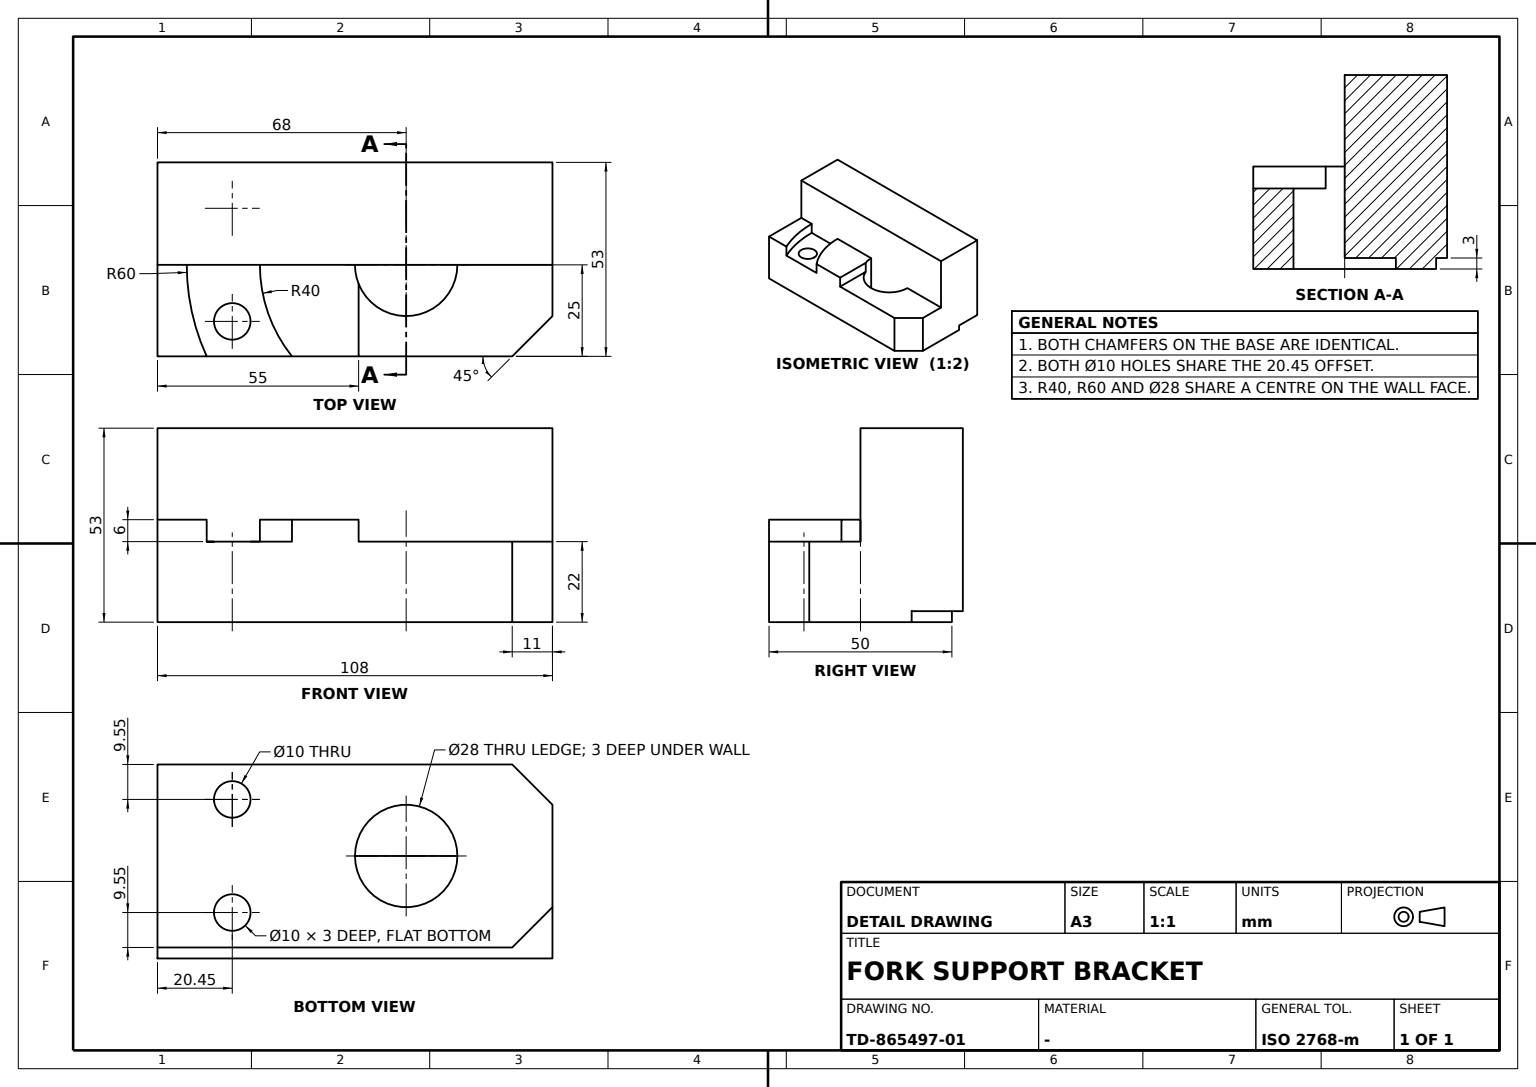
ISO-10303-21;
HEADER;
FILE_DESCRIPTION((''),'2;1');
FILE_NAME('','',(''),(''),'','','');
FILE_SCHEMA(('AUTOMOTIVE_DESIGN'));
ENDSEC;
DATA;
#1=APPLICATION_CONTEXT('');
#2=PRODUCT_CONTEXT('',#1,'mechanical');
#3=PRODUCT('','','',(#2));
#4=PRODUCT_DEFINITION_FORMATION('','',#3);
#5=PRODUCT_DEFINITION_CONTEXT('',#1,'design');
#6=PRODUCT_DEFINITION('','',#4,#5);
#7=PRODUCT_DEFINITION_SHAPE('','',#6);
#8=(LENGTH_UNIT()NAMED_UNIT(*)SI_UNIT(.MILLI.,.METRE.));
#9=(NAMED_UNIT(*)PLANE_ANGLE_UNIT()SI_UNIT($,.RADIAN.));
#10=(NAMED_UNIT(*)SI_UNIT($,.STERADIAN.)SOLID_ANGLE_UNIT());
#11=UNCERTAINTY_MEASURE_WITH_UNIT(LENGTH_MEASURE(1.E-05),#8,'distance_accuracy_value','');
#12=(GEOMETRIC_REPRESENTATION_CONTEXT(3)GLOBAL_UNCERTAINTY_ASSIGNED_CONTEXT((#11))GLOBAL_UNIT_ASSIGNED_CONTEXT((#8,#9,#10))REPRESENTATION_CONTEXT('',''));
#13=CARTESIAN_POINT('',(0.,0.,53.));
#14=VERTEX_POINT('',#13);
#15=CARTESIAN_POINT('',(0.,28.,53.));
#16=VERTEX_POINT('',#15);
#17=CARTESIAN_POINT('',(0.,14.,53.));
#18=DIRECTION('',(0.,1.,0.));
#19=VECTOR('',#18,1000.);
#20=LINE('',#17,#19);
#21=EDGE_CURVE('',#14,#16,#20,.T.);
#22=ORIENTED_EDGE('',*,*,#21,.T.);
#23=CARTESIAN_POINT('',(-108.,28.,53.));
#24=VERTEX_POINT('',#23);
#25=CARTESIAN_POINT('',(-54.,28.,53.));
#26=DIRECTION('',(-1.,0.,0.));
#27=VECTOR('',#26,1000.);
#28=LINE('',#25,#27);
#29=EDGE_CURVE('',#16,#24,#28,.T.);
#30=ORIENTED_EDGE('',*,*,#29,.T.);
#31=CARTESIAN_POINT('',(-108.,0.,53.));
#32=VERTEX_POINT('',#31);
#33=CARTESIAN_POINT('',(-108.,14.,53.));
#34=DIRECTION('',(0.,-1.,0.));
#35=VECTOR('',#34,1000.);
#36=LINE('',#33,#35);
#37=EDGE_CURVE('',#24,#32,#36,.T.);
#38=ORIENTED_EDGE('',*,*,#37,.T.);
#39=CARTESIAN_POINT('',(-54.,0.,53.));
#40=DIRECTION('',(1.,0.,0.));
#41=VECTOR('',#40,1000.);
#42=LINE('',#39,#41);
#43=EDGE_CURVE('',#32,#14,#42,.T.);
#44=ORIENTED_EDGE('',*,*,#43,.T.);
#45=EDGE_LOOP('',(#22,#30,#38,#44));
#46=FACE_OUTER_BOUND('',#45,.T.);
#47=DIRECTION('',(0.,0.,1.));
#48=AXIS2_PLACEMENT_3D('',#15,#47,#26);
#49=PLANE('',#48);
#50=ADVANCED_FACE('',(#46),#49,.T.);
#51=CARTESIAN_POINT('',(-53.,-5.196152,28.));
#52=VERTEX_POINT('',#51);
#53=CARTESIAN_POINT('',(-53.,-25.,28.));
#54=VERTEX_POINT('',#53);
#55=CARTESIAN_POINT('',(-53.,-15.098076,28.));
#56=LINE('',#55,#35);
#57=EDGE_CURVE('',#52,#54,#56,.T.);
#58=ORIENTED_EDGE('',*,*,#57,.F.);
#59=CARTESIAN_POINT('',(-54.,0.,28.));
#60=VERTEX_POINT('',#59);
#61=CARTESIAN_POINT('',(-40.,0.,28.));
#62=AXIS2_PLACEMENT_3D('',#61,#47,#40);
#63=CIRCLE('',#62,14.);
#64=EDGE_CURVE('',#60,#52,#63,.T.);
#65=ORIENTED_EDGE('',*,*,#64,.F.);
#66=CARTESIAN_POINT('',(-80.,0.,28.));
#67=VERTEX_POINT('',#66);
#68=CARTESIAN_POINT('',(-67.,0.,28.));
#69=LINE('',#68,#27);
#70=EDGE_CURVE('',#60,#67,#69,.T.);
#71=ORIENTED_EDGE('',*,*,#70,.T.);
#72=CARTESIAN_POINT('',(-71.22499,-25.,28.));
#73=VERTEX_POINT('',#72);
#74=DIRECTION('',(0.,0.,-1.));
#75=AXIS2_PLACEMENT_3D('',#61,#74,#40);
#76=CIRCLE('',#75,40.);
#77=EDGE_CURVE('',#73,#67,#76,.T.);
#78=ORIENTED_EDGE('',*,*,#77,.F.);
#79=CARTESIAN_POINT('',(-62.112495,-25.,28.));
#80=LINE('',#79,#41);
#81=EDGE_CURVE('',#73,#54,#80,.T.);
#82=ORIENTED_EDGE('',*,*,#81,.T.);
#83=EDGE_LOOP('',(#58,#65,#71,#78,#82));
#84=FACE_OUTER_BOUND('',#83,.T.);
#85=CARTESIAN_POINT('',(0.,0.,28.));
#86=AXIS2_PLACEMENT_3D('',#85,#74,#26);
#87=PLANE('',#86);
#88=ADVANCED_FACE('',(#84),#87,.F.);
#89=CARTESIAN_POINT('',(-108.,25.,3.));
#90=VERTEX_POINT('',#89);
#91=CARTESIAN_POINT('',(-11.,25.,3.));
#92=VERTEX_POINT('',#91);
#93=CARTESIAN_POINT('',(-59.5,25.,3.));
#94=LINE('',#93,#41);
#95=EDGE_CURVE('',#90,#92,#94,.T.);
#96=ORIENTED_EDGE('',*,*,#95,.F.);
#97=CARTESIAN_POINT('',(-108.,28.,3.));
#98=VERTEX_POINT('',#97);
#99=CARTESIAN_POINT('',(-108.,26.5,3.));
#100=LINE('',#99,#35);
#101=EDGE_CURVE('',#98,#90,#100,.T.);
#102=ORIENTED_EDGE('',*,*,#101,.F.);
#103=CARTESIAN_POINT('',(0.,28.,3.));
#104=VERTEX_POINT('',#103);
#105=CARTESIAN_POINT('',(-54.,28.,3.));
#106=LINE('',#105,#27);
#107=EDGE_CURVE('',#104,#98,#106,.T.);
#108=ORIENTED_EDGE('',*,*,#107,.F.);
#109=CARTESIAN_POINT('',(0.,14.,3.));
#110=VERTEX_POINT('',#109);
#111=CARTESIAN_POINT('',(0.,21.,3.));
#112=LINE('',#111,#19);
#113=EDGE_CURVE('',#110,#104,#112,.T.);
#114=ORIENTED_EDGE('',*,*,#113,.F.);
#115=CARTESIAN_POINT('',(-5.5,19.5,3.));
#116=DIRECTION('',(-0.707106781,0.707106781,0.));
#117=VECTOR('',#116,1000.);
#118=LINE('',#115,#117);
#119=EDGE_CURVE('',#110,#92,#118,.T.);
#120=ORIENTED_EDGE('',*,*,#119,.T.);
#121=EDGE_LOOP('',(#96,#102,#108,#114,#120));
#122=FACE_OUTER_BOUND('',#121,.T.);
#123=AXIS2_PLACEMENT_3D('',#103,#47,#26);
#124=PLANE('',#123);
#125=ADVANCED_FACE('',(#122),#124,.F.);
#126=CARTESIAN_POINT('',(-92.552826,15.45085,0.));
#127=VERTEX_POINT('',#126);
#128=CARTESIAN_POINT('',(-82.552826,15.45085,0.));
#129=VERTEX_POINT('',#128);
#130=CARTESIAN_POINT('',(-87.552826,15.45085,0.));
#131=AXIS2_PLACEMENT_3D('',#130,#47,#40);
#132=CIRCLE('',#131,5.);
#133=EDGE_CURVE('',#127,#129,#132,.T.);
#134=ORIENTED_EDGE('',*,*,#133,.T.);
#135=EDGE_CURVE('',#129,#127,#132,.T.);
#136=ORIENTED_EDGE('',*,*,#135,.T.);
#137=EDGE_LOOP('',(#134,#136));
#138=FACE_BOUND('',#137,.T.);
#139=CARTESIAN_POINT('',(-54.,0.,0.));
#140=VERTEX_POINT('',#139);
#141=CARTESIAN_POINT('',(-26.,0.,0.));
#142=VERTEX_POINT('',#141);
#143=CARTESIAN_POINT('',(-40.,0.,0.));
#144=AXIS2_PLACEMENT_3D('',#143,#47,#40);
#145=CIRCLE('',#144,14.);
#146=EDGE_CURVE('',#140,#142,#145,.T.);
#147=ORIENTED_EDGE('',*,*,#146,.T.);
#148=EDGE_CURVE('',#142,#140,#145,.T.);
#149=ORIENTED_EDGE('',*,*,#148,.T.);
#150=EDGE_LOOP('',(#147,#149));
#151=FACE_BOUND('',#150,.T.);
#152=CARTESIAN_POINT('',(-108.,-25.,0.));
#153=VERTEX_POINT('',#152);
#154=CARTESIAN_POINT('',(-108.,25.,0.));
#155=VERTEX_POINT('',#154);
#156=CARTESIAN_POINT('',(-108.,0.,0.));
#157=LINE('',#156,#19);
#158=EDGE_CURVE('',#153,#155,#157,.T.);
#159=ORIENTED_EDGE('',*,*,#158,.T.);
#160=CARTESIAN_POINT('',(-11.,25.,0.));
#161=VERTEX_POINT('',#160);
#162=CARTESIAN_POINT('',(-59.5,25.,0.));
#163=LINE('',#162,#27);
#164=EDGE_CURVE('',#161,#155,#163,.T.);
#165=ORIENTED_EDGE('',*,*,#164,.F.);
#166=CARTESIAN_POINT('',(0.,14.,0.));
#167=VERTEX_POINT('',#166);
#168=CARTESIAN_POINT('',(-5.5,19.5,0.));
#169=LINE('',#168,#117);
#170=EDGE_CURVE('',#167,#161,#169,.T.);
#171=ORIENTED_EDGE('',*,*,#170,.F.);
#172=CARTESIAN_POINT('',(0.,-14.,0.));
#173=VERTEX_POINT('',#172);
#174=CARTESIAN_POINT('',(0.,0.,0.));
#175=LINE('',#174,#19);
#176=EDGE_CURVE('',#173,#167,#175,.T.);
#177=ORIENTED_EDGE('',*,*,#176,.F.);
#178=CARTESIAN_POINT('',(-11.,-25.,0.));
#179=VERTEX_POINT('',#178);
#180=CARTESIAN_POINT('',(-5.5,-19.5,0.));
#181=DIRECTION('',(0.707106781,0.707106781,0.));
#182=VECTOR('',#181,1000.);
#183=LINE('',#180,#182);
#184=EDGE_CURVE('',#179,#173,#183,.T.);
#185=ORIENTED_EDGE('',*,*,#184,.F.);
#186=CARTESIAN_POINT('',(-59.5,-25.,0.));
#187=LINE('',#186,#27);
#188=EDGE_CURVE('',#179,#153,#187,.T.);
#189=ORIENTED_EDGE('',*,*,#188,.T.);
#190=EDGE_LOOP('',(#159,#165,#171,#177,#185,#189));
#191=FACE_OUTER_BOUND('',#190,.T.);
#192=CARTESIAN_POINT('',(-82.552826,-15.45085,0.));
#193=VERTEX_POINT('',#192);
#194=CARTESIAN_POINT('',(-92.552826,-15.45085,0.));
#195=VERTEX_POINT('',#194);
#196=CARTESIAN_POINT('',(-87.552826,-15.45085,0.));
#197=AXIS2_PLACEMENT_3D('',#196,#47,#40);
#198=CIRCLE('',#197,5.);
#199=EDGE_CURVE('',#193,#195,#198,.T.);
#200=ORIENTED_EDGE('',*,*,#199,.T.);
#201=EDGE_CURVE('',#195,#193,#198,.T.);
#202=ORIENTED_EDGE('',*,*,#201,.T.);
#203=EDGE_LOOP('',(#200,#202));
#204=FACE_BOUND('',#203,.T.);
#205=AXIS2_PLACEMENT_3D('',#156,#47,#40);
#206=PLANE('',#205);
#207=ADVANCED_FACE('',(#138,#151,#191,#204),#206,.F.);
#208=ORIENTED_EDGE('',*,*,#95,.T.);
#209=CARTESIAN_POINT('',(-11.,25.,1.5));
#210=VECTOR('',#74,1000.);
#211=LINE('',#209,#210);
#212=EDGE_CURVE('',#92,#161,#211,.T.);
#213=ORIENTED_EDGE('',*,*,#212,.T.);
#214=ORIENTED_EDGE('',*,*,#164,.T.);
#215=CARTESIAN_POINT('',(-108.,25.,1.5));
#216=VECTOR('',#47,1000.);
#217=LINE('',#215,#216);
#218=EDGE_CURVE('',#155,#90,#217,.T.);
#219=ORIENTED_EDGE('',*,*,#218,.T.);
#220=EDGE_LOOP('',(#208,#213,#214,#219));
#221=FACE_OUTER_BOUND('',#220,.T.);
#222=CARTESIAN_POINT('',(0.,25.,0.));
#223=AXIS2_PLACEMENT_3D('',#222,#18,#26);
#224=PLANE('',#223);
#225=ADVANCED_FACE('',(#221),#224,.T.);
#226=CARTESIAN_POINT('',(-82.552826,15.45085,3.));
#227=VERTEX_POINT('',#226);
#228=CARTESIAN_POINT('',(-92.552826,15.45085,3.));
#229=VERTEX_POINT('',#228);
#230=CARTESIAN_POINT('',(-87.552826,15.45085,3.));
#231=AXIS2_PLACEMENT_3D('',#230,#47,#26);
#232=CIRCLE('',#231,5.);
#233=EDGE_CURVE('',#227,#229,#232,.T.);
#234=ORIENTED_EDGE('',*,*,#233,.T.);
#235=CARTESIAN_POINT('',(-92.552826,15.45085,10.34));
#236=LINE('',#235,#210);
#237=EDGE_CURVE('',#229,#127,#236,.T.);
#238=ORIENTED_EDGE('',*,*,#237,.T.);
#239=ORIENTED_EDGE('',*,*,#135,.F.);
#240=CARTESIAN_POINT('',(-82.552826,15.45085,10.34));
#241=LINE('',#240,#210);
#242=EDGE_CURVE('',#227,#129,#241,.T.);
#243=ORIENTED_EDGE('',*,*,#242,.F.);
#244=EDGE_LOOP('',(#234,#238,#239,#243));
#245=FACE_OUTER_BOUND('',#244,.T.);
#246=CARTESIAN_POINT('',(-87.552826,15.45085,10.34));
#247=AXIS2_PLACEMENT_3D('',#246,#74,#40);
#248=CYLINDRICAL_SURFACE('',#247,5.);
#249=ADVANCED_FACE('',(#245),#248,.F.);
#250=CARTESIAN_POINT('',(-26.,0.,3.));
#251=VERTEX_POINT('',#250);
#252=CARTESIAN_POINT('',(-54.,0.,3.));
#253=VERTEX_POINT('',#252);
#254=CARTESIAN_POINT('',(-40.,0.,3.));
#255=AXIS2_PLACEMENT_3D('',#254,#47,#26);
#256=CIRCLE('',#255,14.);
#257=EDGE_CURVE('',#251,#253,#256,.T.);
#258=ORIENTED_EDGE('',*,*,#257,.F.);
#259=LINE('',#254,#41);
#260=EDGE_CURVE('',#253,#251,#259,.T.);
#261=ORIENTED_EDGE('',*,*,#260,.F.);
#262=EDGE_LOOP('',(#258,#261));
#263=FACE_OUTER_BOUND('',#262,.T.);
#264=ADVANCED_FACE('',(#263),#124,.F.);
#265=CARTESIAN_POINT('',(-53.,-25.,22.));
#266=VERTEX_POINT('',#265);
#267=CARTESIAN_POINT('',(-53.,-25.,25.));
#268=LINE('',#267,#210);
#269=EDGE_CURVE('',#54,#266,#268,.T.);
#270=ORIENTED_EDGE('',*,*,#269,.F.);
#271=ORIENTED_EDGE('',*,*,#81,.F.);
#272=CARTESIAN_POINT('',(-71.22499,-25.,22.));
#273=VERTEX_POINT('',#272);
#274=CARTESIAN_POINT('',(-71.22499,-25.,25.));
#275=LINE('',#274,#210);
#276=EDGE_CURVE('',#73,#273,#275,.T.);
#277=ORIENTED_EDGE('',*,*,#276,.T.);
#278=CARTESIAN_POINT('',(-94.543561,-25.,22.));
#279=VERTEX_POINT('',#278);
#280=CARTESIAN_POINT('',(-82.884275,-25.,22.));
#281=LINE('',#280,#41);
#282=EDGE_CURVE('',#279,#273,#281,.T.);
#283=ORIENTED_EDGE('',*,*,#282,.F.);
#284=CARTESIAN_POINT('',(-94.543561,-25.,28.));
#285=VERTEX_POINT('',#284);
#286=CARTESIAN_POINT('',(-94.543561,-25.,25.));
#287=LINE('',#286,#210);
#288=EDGE_CURVE('',#285,#279,#287,.T.);
#289=ORIENTED_EDGE('',*,*,#288,.F.);
#290=CARTESIAN_POINT('',(-108.,-25.,28.));
#291=VERTEX_POINT('',#290);
#292=CARTESIAN_POINT('',(-101.27178,-25.,28.));
#293=LINE('',#292,#41);
#294=EDGE_CURVE('',#291,#285,#293,.T.);
#295=ORIENTED_EDGE('',*,*,#294,.F.);
#296=CARTESIAN_POINT('',(-108.,-25.,14.));
#297=LINE('',#296,#216);
#298=EDGE_CURVE('',#153,#291,#297,.T.);
#299=ORIENTED_EDGE('',*,*,#298,.F.);
#300=ORIENTED_EDGE('',*,*,#188,.F.);
#301=CARTESIAN_POINT('',(-11.,-25.,22.));
#302=VERTEX_POINT('',#301);
#303=CARTESIAN_POINT('',(-11.,-25.,11.));
#304=LINE('',#303,#210);
#305=EDGE_CURVE('',#302,#179,#304,.T.);
#306=ORIENTED_EDGE('',*,*,#305,.F.);
#307=CARTESIAN_POINT('',(-32.,-25.,22.));
#308=LINE('',#307,#41);
#309=EDGE_CURVE('',#266,#302,#308,.T.);
#310=ORIENTED_EDGE('',*,*,#309,.F.);
#311=EDGE_LOOP('',(#270,#271,#277,#283,#289,#295,#299,#300,#306,#310));
#312=FACE_OUTER_BOUND('',#311,.T.);
#313=CARTESIAN_POINT('',(0.,-25.,0.));
#314=AXIS2_PLACEMENT_3D('',#313,#18,#26);
#315=PLANE('',#314);
#316=ADVANCED_FACE('',(#312),#315,.F.);
#317=CARTESIAN_POINT('',(0.,-14.,22.));
#318=VERTEX_POINT('',#317);
#319=CARTESIAN_POINT('',(0.,-14.,11.));
#320=LINE('',#319,#210);
#321=EDGE_CURVE('',#318,#173,#320,.T.);
#322=ORIENTED_EDGE('',*,*,#321,.F.);
#323=CARTESIAN_POINT('',(-5.5,-19.5,22.));
#324=DIRECTION('',(-0.707106781,-0.707106781,0.));
#325=VECTOR('',#324,1000.);
#326=LINE('',#323,#325);
#327=EDGE_CURVE('',#318,#302,#326,.T.);
#328=ORIENTED_EDGE('',*,*,#327,.T.);
#329=ORIENTED_EDGE('',*,*,#305,.T.);
#330=ORIENTED_EDGE('',*,*,#184,.T.);
#331=EDGE_LOOP('',(#322,#328,#329,#330));
#332=FACE_OUTER_BOUND('',#331,.T.);
#333=CARTESIAN_POINT('',(-11.,-25.,-5.6));
#334=AXIS2_PLACEMENT_3D('',#333,#116,#47);
#335=PLANE('',#334);
#336=ADVANCED_FACE('',(#332),#335,.F.);
#337=ORIENTED_EDGE('',*,*,#242,.T.);
#338=ORIENTED_EDGE('',*,*,#133,.F.);
#339=ORIENTED_EDGE('',*,*,#237,.F.);
#340=EDGE_CURVE('',#229,#227,#232,.T.);
#341=ORIENTED_EDGE('',*,*,#340,.T.);
#342=EDGE_LOOP('',(#337,#338,#339,#341));
#343=FACE_OUTER_BOUND('',#342,.T.);
#344=ADVANCED_FACE('',(#343),#248,.F.);
#345=CARTESIAN_POINT('',(-100.,0.,22.));
#346=VERTEX_POINT('',#345);
#347=CARTESIAN_POINT('',(-100.,0.,28.));
#348=VERTEX_POINT('',#347);
#349=CARTESIAN_POINT('',(-100.,0.,25.));
#350=LINE('',#349,#216);
#351=EDGE_CURVE('',#346,#348,#350,.T.);
#352=ORIENTED_EDGE('',*,*,#351,.T.);
#353=CIRCLE('',#62,60.);
#354=EDGE_CURVE('',#348,#285,#353,.T.);
#355=ORIENTED_EDGE('',*,*,#354,.T.);
#356=ORIENTED_EDGE('',*,*,#288,.T.);
#357=CARTESIAN_POINT('',(-40.,0.,22.));
#358=AXIS2_PLACEMENT_3D('',#357,#47,#40);
#359=CIRCLE('',#358,60.);
#360=EDGE_CURVE('',#346,#279,#359,.T.);
#361=ORIENTED_EDGE('',*,*,#360,.F.);
#362=EDGE_LOOP('',(#352,#355,#356,#361));
#363=FACE_OUTER_BOUND('',#362,.T.);
#364=CARTESIAN_POINT('',(-40.,0.,25.));
#365=AXIS2_PLACEMENT_3D('',#364,#74,#40);
#366=CYLINDRICAL_SURFACE('',#365,60.);
#367=ADVANCED_FACE('',(#363),#366,.F.);
#368=CARTESIAN_POINT('',(-82.552826,-15.45085,22.));
#369=VERTEX_POINT('',#368);
#370=CARTESIAN_POINT('',(-82.552826,-15.45085,10.34));
#371=LINE('',#370,#210);
#372=EDGE_CURVE('',#369,#193,#371,.T.);
#373=ORIENTED_EDGE('',*,*,#372,.F.);
#374=CARTESIAN_POINT('',(-92.552826,-15.45085,22.));
#375=VERTEX_POINT('',#374);
#376=CARTESIAN_POINT('',(-87.552826,-15.45085,22.));
#377=AXIS2_PLACEMENT_3D('',#376,#47,#40);
#378=CIRCLE('',#377,5.);
#379=EDGE_CURVE('',#369,#375,#378,.T.);
#380=ORIENTED_EDGE('',*,*,#379,.T.);
#381=CARTESIAN_POINT('',(-92.552826,-15.45085,10.34));
#382=LINE('',#381,#210);
#383=EDGE_CURVE('',#375,#195,#382,.T.);
#384=ORIENTED_EDGE('',*,*,#383,.T.);
#385=ORIENTED_EDGE('',*,*,#199,.F.);
#386=EDGE_LOOP('',(#373,#380,#384,#385));
#387=FACE_OUTER_BOUND('',#386,.T.);
#388=CARTESIAN_POINT('',(-87.552826,-15.45085,10.34));
#389=AXIS2_PLACEMENT_3D('',#388,#74,#40);
#390=CYLINDRICAL_SURFACE('',#389,5.);
#391=ADVANCED_FACE('',(#387),#390,.F.);
#392=CARTESIAN_POINT('',(-26.,0.,22.));
#393=VERTEX_POINT('',#392);
#394=CARTESIAN_POINT('',(-53.,-5.196152,22.));
#395=VERTEX_POINT('',#394);
#396=AXIS2_PLACEMENT_3D('',#357,#74,#40);
#397=CIRCLE('',#396,14.);
#398=EDGE_CURVE('',#393,#395,#397,.T.);
#399=ORIENTED_EDGE('',*,*,#398,.F.);
#400=CARTESIAN_POINT('',(-26.,0.,12.5));
#401=LINE('',#400,#210);
#402=EDGE_CURVE('',#393,#251,#401,.T.);
#403=ORIENTED_EDGE('',*,*,#402,.T.);
#404=CARTESIAN_POINT('',(-26.,0.,14.));
#405=LINE('',#404,#210);
#406=EDGE_CURVE('',#251,#142,#405,.T.);
#407=ORIENTED_EDGE('',*,*,#406,.T.);
#408=ORIENTED_EDGE('',*,*,#146,.F.);
#409=CARTESIAN_POINT('',(-54.,0.,14.));
#410=LINE('',#409,#210);
#411=EDGE_CURVE('',#253,#140,#410,.T.);
#412=ORIENTED_EDGE('',*,*,#411,.F.);
#413=CARTESIAN_POINT('',(-54.,0.,15.5));
#414=LINE('',#413,#210);
#415=EDGE_CURVE('',#60,#253,#414,.T.);
#416=ORIENTED_EDGE('',*,*,#415,.F.);
#417=ORIENTED_EDGE('',*,*,#64,.T.);
#418=CARTESIAN_POINT('',(-53.,-5.196152,14.));
#419=LINE('',#418,#210);
#420=EDGE_CURVE('',#52,#395,#419,.T.);
#421=ORIENTED_EDGE('',*,*,#420,.T.);
#422=EDGE_LOOP('',(#399,#403,#407,#408,#412,#416,#417,#421));
#423=FACE_OUTER_BOUND('',#422,.T.);
#424=CARTESIAN_POINT('',(-40.,0.,13.34));
#425=AXIS2_PLACEMENT_3D('',#424,#74,#40);
#426=CYLINDRICAL_SURFACE('',#425,14.);
#427=ADVANCED_FACE('',(#423),#426,.F.);
#428=ORIENTED_EDGE('',*,*,#351,.F.);
#429=CARTESIAN_POINT('',(-80.,0.,22.));
#430=VERTEX_POINT('',#429);
#431=CARTESIAN_POINT('',(-90.,0.,22.));
#432=LINE('',#431,#41);
#433=EDGE_CURVE('',#346,#430,#432,.T.);
#434=ORIENTED_EDGE('',*,*,#433,.T.);
#435=CARTESIAN_POINT('',(-80.,0.,25.));
#436=LINE('',#435,#216);
#437=EDGE_CURVE('',#430,#67,#436,.T.);
#438=ORIENTED_EDGE('',*,*,#437,.T.);
#439=ORIENTED_EDGE('',*,*,#70,.F.);
#440=ORIENTED_EDGE('',*,*,#415,.T.);
#441=ORIENTED_EDGE('',*,*,#260,.T.);
#442=ORIENTED_EDGE('',*,*,#402,.F.);
#443=CARTESIAN_POINT('',(0.,0.,22.));
#444=VERTEX_POINT('',#443);
#445=CARTESIAN_POINT('',(-13.,0.,22.));
#446=LINE('',#445,#27);
#447=EDGE_CURVE('',#444,#393,#446,.T.);
#448=ORIENTED_EDGE('',*,*,#447,.F.);
#449=CARTESIAN_POINT('',(0.,0.,37.5));
#450=LINE('',#449,#216);
#451=EDGE_CURVE('',#444,#14,#450,.T.);
#452=ORIENTED_EDGE('',*,*,#451,.T.);
#453=ORIENTED_EDGE('',*,*,#43,.F.);
#454=CARTESIAN_POINT('',(-108.,0.,28.));
#455=VERTEX_POINT('',#454);
#456=CARTESIAN_POINT('',(-108.,0.,40.5));
#457=LINE('',#456,#216);
#458=EDGE_CURVE('',#455,#32,#457,.T.);
#459=ORIENTED_EDGE('',*,*,#458,.F.);
#460=CARTESIAN_POINT('',(-104.,0.,28.));
#461=LINE('',#460,#41);
#462=EDGE_CURVE('',#455,#348,#461,.T.);
#463=ORIENTED_EDGE('',*,*,#462,.T.);
#464=EDGE_LOOP('',(#428,#434,#438,#439,#440,#441,#442,#448,#452,#453,#459,#463));
#465=FACE_OUTER_BOUND('',#464,.T.);
#466=AXIS2_PLACEMENT_3D('',#85,#18,#26);
#467=PLANE('',#466);
#468=ADVANCED_FACE('',(#465),#467,.F.);
#469=CARTESIAN_POINT('',(0.,-7.,22.));
#470=LINE('',#469,#19);
#471=EDGE_CURVE('',#318,#444,#470,.T.);
#472=ORIENTED_EDGE('',*,*,#471,.F.);
#473=ORIENTED_EDGE('',*,*,#321,.T.);
#474=ORIENTED_EDGE('',*,*,#176,.T.);
#475=CARTESIAN_POINT('',(0.,14.,1.5));
#476=LINE('',#475,#210);
#477=EDGE_CURVE('',#110,#167,#476,.T.);
#478=ORIENTED_EDGE('',*,*,#477,.F.);
#479=ORIENTED_EDGE('',*,*,#113,.T.);
#480=CARTESIAN_POINT('',(0.,28.,28.));
#481=LINE('',#480,#216);
#482=EDGE_CURVE('',#104,#16,#481,.T.);
#483=ORIENTED_EDGE('',*,*,#482,.T.);
#484=ORIENTED_EDGE('',*,*,#21,.F.);
#485=ORIENTED_EDGE('',*,*,#451,.F.);
#486=EDGE_LOOP('',(#472,#473,#474,#478,#479,#483,#484,#485));
#487=FACE_OUTER_BOUND('',#486,.T.);
#488=AXIS2_PLACEMENT_3D('',#174,#26,#47);
#489=PLANE('',#488);
#490=ADVANCED_FACE('',(#487),#489,.F.);
#491=EDGE_CURVE('',#375,#369,#378,.T.);
#492=ORIENTED_EDGE('',*,*,#491,.T.);
#493=ORIENTED_EDGE('',*,*,#372,.T.);
#494=ORIENTED_EDGE('',*,*,#201,.F.);
#495=ORIENTED_EDGE('',*,*,#383,.F.);
#496=EDGE_LOOP('',(#492,#493,#494,#495));
#497=FACE_OUTER_BOUND('',#496,.T.);
#498=ADVANCED_FACE('',(#497),#390,.F.);
#499=ORIENTED_EDGE('',*,*,#379,.F.);
#500=ORIENTED_EDGE('',*,*,#491,.F.);
#501=EDGE_LOOP('',(#499,#500));
#502=FACE_BOUND('',#501,.T.);
#503=ORIENTED_EDGE('',*,*,#360,.T.);
#504=ORIENTED_EDGE('',*,*,#282,.T.);
#505=CIRCLE('',#396,40.);
#506=EDGE_CURVE('',#273,#430,#505,.T.);
#507=ORIENTED_EDGE('',*,*,#506,.T.);
#508=ORIENTED_EDGE('',*,*,#433,.F.);
#509=EDGE_LOOP('',(#503,#504,#507,#508));
#510=FACE_OUTER_BOUND('',#509,.T.);
#511=CARTESIAN_POINT('',(0.,-11.,22.));
#512=AXIS2_PLACEMENT_3D('',#511,#47,#18);
#513=PLANE('',#512);
#514=ADVANCED_FACE('',(#502,#510),#513,.T.);
#515=ORIENTED_EDGE('',*,*,#354,.F.);
#516=ORIENTED_EDGE('',*,*,#462,.F.);
#517=CARTESIAN_POINT('',(-108.,-12.5,28.));
#518=LINE('',#517,#19);
#519=EDGE_CURVE('',#291,#455,#518,.T.);
#520=ORIENTED_EDGE('',*,*,#519,.F.);
#521=ORIENTED_EDGE('',*,*,#294,.T.);
#522=EDGE_LOOP('',(#515,#516,#520,#521));
#523=FACE_OUTER_BOUND('',#522,.T.);
#524=ADVANCED_FACE('',(#523),#87,.F.);
#525=ORIENTED_EDGE('',*,*,#506,.F.);
#526=ORIENTED_EDGE('',*,*,#276,.F.);
#527=ORIENTED_EDGE('',*,*,#77,.T.);
#528=ORIENTED_EDGE('',*,*,#437,.F.);
#529=EDGE_LOOP('',(#525,#526,#527,#528));
#530=FACE_OUTER_BOUND('',#529,.T.);
#531=CYLINDRICAL_SURFACE('',#365,40.);
#532=ADVANCED_FACE('',(#530),#531,.T.);
#533=ORIENTED_EDGE('',*,*,#340,.F.);
#534=ORIENTED_EDGE('',*,*,#233,.F.);
#535=EDGE_LOOP('',(#533,#534));
#536=FACE_OUTER_BOUND('',#535,.T.);
#537=ADVANCED_FACE('',(#536),#124,.F.);
#538=CARTESIAN_POINT('',(-53.,-15.098076,22.));
#539=LINE('',#538,#35);
#540=EDGE_CURVE('',#395,#266,#539,.T.);
#541=ORIENTED_EDGE('',*,*,#540,.F.);
#542=ORIENTED_EDGE('',*,*,#420,.F.);
#543=ORIENTED_EDGE('',*,*,#57,.T.);
#544=ORIENTED_EDGE('',*,*,#269,.T.);
#545=EDGE_LOOP('',(#541,#542,#543,#544));
#546=FACE_OUTER_BOUND('',#545,.T.);
#547=CARTESIAN_POINT('',(-53.,25.,28.));
#548=AXIS2_PLACEMENT_3D('',#547,#40,#34);
#549=PLANE('',#548);
#550=ADVANCED_FACE('',(#546),#549,.T.);
#551=ORIENTED_EDGE('',*,*,#406,.F.);
#552=ORIENTED_EDGE('',*,*,#257,.T.);
#553=ORIENTED_EDGE('',*,*,#411,.T.);
#554=ORIENTED_EDGE('',*,*,#148,.F.);
#555=EDGE_LOOP('',(#551,#552,#553,#554));
#556=FACE_OUTER_BOUND('',#555,.T.);
#557=ADVANCED_FACE('',(#556),#426,.F.);
#558=ORIENTED_EDGE('',*,*,#37,.F.);
#559=CARTESIAN_POINT('',(-108.,28.,28.));
#560=LINE('',#559,#216);
#561=EDGE_CURVE('',#98,#24,#560,.T.);
#562=ORIENTED_EDGE('',*,*,#561,.F.);
#563=ORIENTED_EDGE('',*,*,#101,.T.);
#564=ORIENTED_EDGE('',*,*,#218,.F.);
#565=ORIENTED_EDGE('',*,*,#158,.F.);
#566=ORIENTED_EDGE('',*,*,#298,.T.);
#567=ORIENTED_EDGE('',*,*,#519,.T.);
#568=ORIENTED_EDGE('',*,*,#458,.T.);
#569=EDGE_LOOP('',(#558,#562,#563,#564,#565,#566,#567,#568));
#570=FACE_OUTER_BOUND('',#569,.T.);
#571=AXIS2_PLACEMENT_3D('',#454,#40,#74);
#572=PLANE('',#571);
#573=ADVANCED_FACE('',(#570),#572,.F.);
#574=ORIENTED_EDGE('',*,*,#447,.T.);
#575=ORIENTED_EDGE('',*,*,#398,.T.);
#576=ORIENTED_EDGE('',*,*,#540,.T.);
#577=ORIENTED_EDGE('',*,*,#309,.T.);
#578=ORIENTED_EDGE('',*,*,#327,.F.);
#579=ORIENTED_EDGE('',*,*,#471,.T.);
#580=EDGE_LOOP('',(#574,#575,#576,#577,#578,#579));
#581=FACE_OUTER_BOUND('',#580,.T.);
#582=ADVANCED_FACE('',(#581),#513,.T.);
#583=ORIENTED_EDGE('',*,*,#482,.F.);
#584=ORIENTED_EDGE('',*,*,#107,.T.);
#585=ORIENTED_EDGE('',*,*,#561,.T.);
#586=ORIENTED_EDGE('',*,*,#29,.F.);
#587=EDGE_LOOP('',(#583,#584,#585,#586));
#588=FACE_OUTER_BOUND('',#587,.T.);
#589=AXIS2_PLACEMENT_3D('',#559,#34,#40);
#590=PLANE('',#589);
#591=ADVANCED_FACE('',(#588),#590,.F.);
#592=ORIENTED_EDGE('',*,*,#170,.T.);
#593=ORIENTED_EDGE('',*,*,#212,.F.);
#594=ORIENTED_EDGE('',*,*,#119,.F.);
#595=ORIENTED_EDGE('',*,*,#477,.T.);
#596=EDGE_LOOP('',(#592,#593,#594,#595));
#597=FACE_OUTER_BOUND('',#596,.T.);
#598=CARTESIAN_POINT('',(0.,14.,33.6));
#599=AXIS2_PLACEMENT_3D('',#598,#181,#74);
#600=PLANE('',#599);
#601=ADVANCED_FACE('',(#597),#600,.T.);
#602=CLOSED_SHELL('',(#50,#88,#125,#207,#225,#249,#264,#316,#336,#344,#367,#391,#427,#468,#490,#498,#514,#524,#532,#537,#550,#557,#573,#582,#591,#601));
#603=MANIFOLD_SOLID_BREP('',#602);
#604=ADVANCED_BREP_SHAPE_REPRESENTATION('',(#603),#12);
#605=SHAPE_DEFINITION_REPRESENTATION(#7,#604);
ENDSEC;
END-ISO-10303-21;
